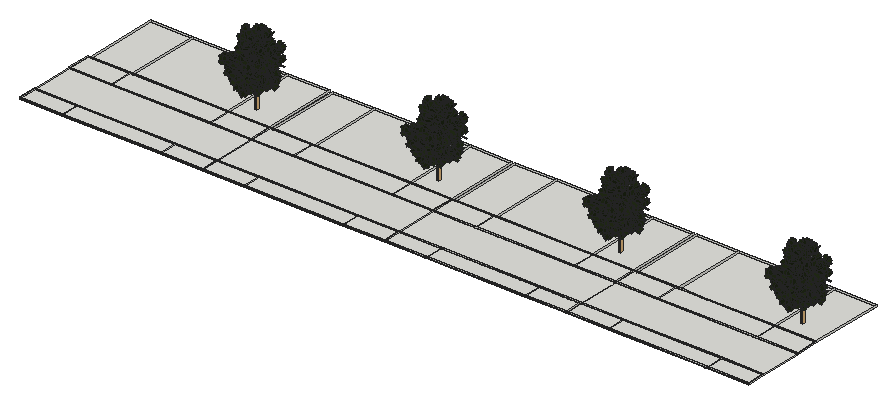
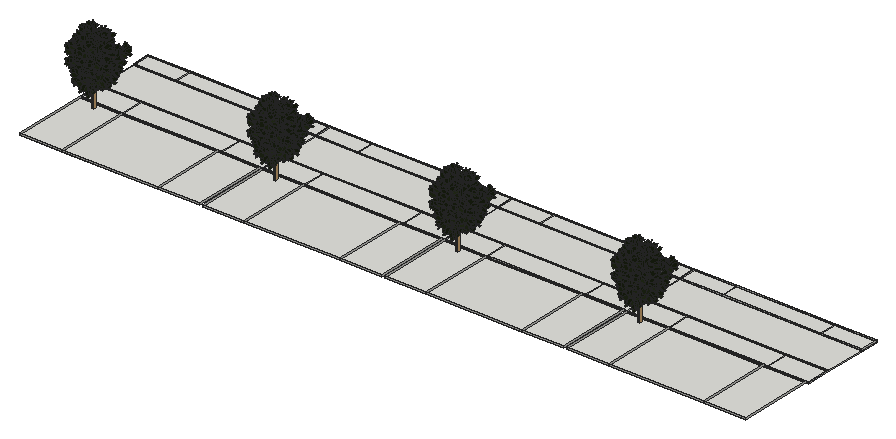
# SketchUp Ruby script. Lengths in inches.
U = 1.inch
M = Sketchup.active_model
def pt(a) = Geom::Point3d.new(a.map { |v| v * U })
def face(e, loops, mat)
  f = e.add_face(loops[0].map { |a| pt(a) })
  loops[1..].each { |l| e.add_face(l.map { |a| pt(a) }).erase! }
  f.material = f.back_material = mat if mat
  f
end
# faces: each face lists its corners as indices into pts; further lists are holes
def faces(e, pts, list, mat = nil) = list.each { |f| face(e, (f[0].is_a?(Array) ? f : [f]).map { |l| l.map { |i| pts[i] } }, mat) }
# xy, xz, yz: faces in a plane at the given z, y or x. An outline is a flat list of corners, or four numbers for a rectangle; further outlines are holes
def ring(l) = l.size == 4 ? [[l[0], l[1]], [l[2], l[1]], [l[2], l[3]], [l[0], l[3]]] : l.each_slice(2).to_a
def flat(e, list, mat, &to3) = list.each { |f| face(e, (f[0].is_a?(Array) ? f : [f]).map { |l| ring(l).map { |u, v| to3.(u, v) } }, mat) }
def xy(e, z, list, mat = nil) = flat(e, list, mat) { |x, y| [x, y, z] }
def xz(e, y, list, mat = nil) = flat(e, list, mat) { |x, z| [x, y, z] }
def yz(e, x, list, mat = nil) = flat(e, list, mat) { |y, z| [x, y, z] }
def lines(e, pts, list) = list.each { |a, b| e.add_line(pt(pts[a]), pt(pts[b])) }
# prism: a flat outline (further loops are holes) pulled along v
def prism(e, loops, v, mat = nil)
  f = face(e, loops, mat); d = Geom::Vector3d.new(v.map { |x| x * U })
  f.pushpull(f.normal.samedirection?(d) ? d.length : -d.length)
end
def box(e, o, s, mat = nil) = prism(e, [[o, [o[0] + s[0], o[1], o[2]], [o[0] + s[0], o[1] + s[1], o[2]], [o[0], o[1] + s[1], o[2]]]], [0, 0, s[2]], mat)
def at(x, y, z, deg = 0) = Geom::Transformation.translation(pt([x, y, z])) * Geom::Transformation.rotation(ORIGIN, Z_AXIS, deg.degrees)
def axes(o, x, y, z) = Geom::Transformation.new([*x, 0, *y, 0, *z, 0, *pt(o).to_a, 1])
def part(name) = M.definitions.add(name)
# library, detail: a bought-in or finely detailed component or shape, given as its bounding box
def library(name, o, s) = part(name).tap { |d| box(d.entities, o, s) }
def detail(e, o, s) = box(e.add_group.entities, o, s)
def put(e, d, t, mat = nil) = e.add_instance(d, t).tap { |i| i.material = mat if mat }
def group(e, t, mat = nil) = e.add_group.tap { |g| g.transformation = t; g.material = mat if mat }.entities
root = M.entities
M.materials.add("Green ash – green texture").color = [33, 41, 22]
M.materials.add("[Color_005]").color = [114, 114, 114]
M.materials.add("[Color_D09]1").color = [86, 59, 49]
c1 = part("Component\#31")
xz(c1.entities,0,[[2.54,0,9.87,0.64,10.99,2.07,11.4,3.42,15.13,2.28,14.48,4.31,16.14,5.21,16.14,6.08,19.81,7.28,19.6,9.67,17.45,11.49,17.45,12.16,18.82,14.37,17.48,14.37,14.41,13.66,14.41,15.23,12.5625,17.49,9.84,15.21,8.9,13.85,7.74,13.625,7.35,12.68,6.87,13.02,6.35,12.27,5.92,10.47,4.2,7.42,2.84,6.89,0,2.38,0.07,1.59,2.8125,4.94,3.37,3.59,2.54,3.37,2.12,2.22]],"Green ash – green texture")
c2 = part("Component\#30")
xz(c2.entities,0,[[1.1,0,1.61,0,2.73,1.11,4.34,2.72,5.21,6.36,5.85,7.16,6.35,6.9375,6.85,8.05,8.03,8.05,8.625,9.25,10.11,11.7,9.56,13.83,9.56,15.84,7.83,15.84,6.03,14.37,5.31,16.54,4.4375,17.39,1.45,14.31,0,9.15,1.4,5.18,3.01,6.08,1.98,1.39]],"Green ash – green texture")
c3 = part("Component\#32")
put(c3.entities,c1,axes([0,7.77,0],[1,0,0],[0,0.89571,0.44464],[0,-0.44464,0.89571]))
put(c3.entities,c2,axes([2.15,6.37,5.26],[0.57629,-0.80824,0.12095],[0.79263,0.51673,-0.3236],[0.19905,0.28236,0.93843]))
c4 = part("Component\#33")
put(c4.entities,c3,axes([-4.97,-3.22,4.05],[0.69883,-0.69034,0.18725],[0.53248,0.3273,-0.7806],[0.47759,0.64522,0.59632]))
c5 = part("Component\#34")
put(c5.entities,c4,axes([0,5.2,2.2],[1,0,0],[0,0.90259,0.43051],[0,-0.43051,0.90259]))
c6 = part("leaf group 2")
put(c6.entities,c5,axes([-11.99,4.41,-4.35],[2.22014,-0.82385,1.14017],[1.36501,1.77637,-1.37441],[-0.33979,1.75315,1.92841]))
c7 = part("Component\#37")
put(c7.entities,c6,axes([-5.27,11.65,1.68],[-0.48323,0.10636,-0.43072],[-0.11515,-0.64511,-0.03012],[-0.42845,0.05342,0.49388]))
c8 = part("Component\#36")
xz(c8.entities,0,[[0.64,0,0,0.1875,4.21,2.81,8.59,4.11,12.8,4.11,19.57,2.81,12.8,3.73,8.59,3.73,4.21,2.3125]],"[Color_D09]1")
c9 = part("Leaf cluster \#1")
put(c9.entities,c7,axes([23.53,12.57,24.85],[0.06536,-0.90475,-0.42089],[0.61791,-0.2945,0.72901],[-0.78353,-0.30772,0.53981]))
put(c9.entities,c7,axes([22.7,12.25,24.83],[-0.47146,-0.89493,0.11311],[0.80135,-0.48549,-0.35888],[0.36776,-0.0521,0.90651]))
put(c9.entities,c7,axes([24.25,0.65,20.83],[0.8253,-0.50372,0.24924],[0.23848,0.71461,0.65749],[-0.51157,-0.48438,0.71194]))
put(c9.entities,c7,axes([23.54,-2.45,18.63],[0.04689,-0.92492,0.3511],[0.72122,-0.28285,-0.64421],[0.71641,0.2674,0.65188]))
put(c9.entities,c7,axes([22.39,16.15,27.04],[-0.5311,-0.82173,0.2419],[0.41574,0.01583,0.89559],[-0.77461,0.50499,0.40813]))
put(c9.entities,c8,axes([22.76,-5.09,13.48],[0,1.66539,0.44624],[-1.72414,0,0],[0,-0.44624,1.66539]))
c10 = part("Component\#35")
p = [[0,0,0.13],[0.41,0.77,0],[4.07,2.79,10.125],[3.73,2.15,10.23],[7.66,4.77,23.875],[7.4,4.27,23.96],
  [8.6875,5.26,35.99],[8.5,4.91,36.05],[8.32,4.9375,46.95],[8.21,4.74,46.98]]
faces(c10.entities,p,[[0,1,2,3],[3,2,4,5],[4,6,7,5],[6,8,9,7]],"[Color_005]")
c11 = part("Component\#39")
put(c11.entities,c10,axes([3.13,0.17,-0.45],[3.38032,6.88592,0.52481],[-5.85488,3.97559,0.303],[0,-1.35912,3.54524]))
put(c11.entities,c7,axes([0.37,31.375,148.94],[0.47772,0.64064,-1.51139],[2.85768,-0.62659,0.20284],[-0.43926,-3.3797,-0.3241]))
c12 = part("Leafy branch \#1")
put(c12.entities,c9,axes([28.11,72.66,46.26],[0.77413,-0.41274,-0.47998],[0.6311,0.56229,0.53435],[0.04934,-0.71657,0.69577]))
put(c12.entities,c9,axes([31.25,3.94,9.17],[0.73236,0.67893,0.05208],[-0.46223,0.55185,-0.69413],[-0.5,0.48428,0.71797]))
put(c12.entities,c9,axes([20.16,84.84,57.95],[0.96628,0.19619,0.16678],[-0.2575,0.73909,0.62245],[-0.00115,-0.6444,0.76469]))
put(c12.entities,c9,axes([30.13,29.18,11.93],[0.86603,0.2796,0.41452],[0,0.82904,-0.55919],[-0.5,0.48428,0.71797]))
put(c12.entities,c9,axes([47.67,28.63,-3.7],[0.1205,-0.71255,0.69119],[0.96646,0.24327,0.08231],[-0.2268,0.65809,0.71797]))
put(c12.entities,c9,axes([48.76,50.64,76.31],[-0.6716,0.46861,-0.57389],[0.01402,0.78248,0.62252],[0.74078,0.41004,-0.53209]))
put(c12.entities,c11,axes([42.34,0,10.34],[0.39368,0,0],[0,0.22544,-0.24092],[0,0.54032,0.50562]))
put(c12.entities,c9,axes([64.51,80.82,101.08],[-0.99604,0.06562,-0.06004],[-0.0106,0.58266,0.81265],[0.08831,0.81006,-0.57966]))
c13 = library("Component\#40",[-6.35,9.4375,-76.57],[12.56,13.68,315.77])
c14 = part("Component\#43")
put(c14.entities,c9,axes([-3.64,36.17,23.18],[0.95801,0.10249,0.26779],[-0.28581,0.41631,0.86313],[-0.02302,-0.90343,0.42812]))
put(c14.entities,c9,axes([13.16,55.79,39.92],[0.70711,-0.61725,0.34497],[0,0.48786,0.87292],[-0.70711,-0.61725,0.34497]))
put(c14.entities,c11,axes([18.8125,5.17,0.46],[0.25503,0,0],[0,0.20007,-0.0752],[0,0.16866,0.44872]))
put(c14.entities,c9,axes([23.62,-10.17,21.5],[-0.56253,0.81775,0.12181],[0.38738,0.13053,0.91263],[0.73041,0.56057,-0.39021]))
put(c14.entities,c9,axes([45.18,27.18,68.96],[-0.96593,-0.22593,0.12627],[0.12295,0.02876,0.992],[-0.22775,0.97372,0]))
c15 = part("Component\#42")
put(c15.entities,c11,axes([21.47,3.93,0.22],[0.25503,0,0],[0,0.21068,-0.03601],[0,0.08077,0.47252]))
put(c15.entities,c9,axes([-4.05,13.6875,55.34],[0.70711,0.70373,-0.069],[0,0.09758,0.99523],[0.70711,-0.70373,0.069]))
put(c15.entities,c9,axes([6.52,33.54,18.07],[0.92587,-0.37604,0.03687],[0,0.09758,0.99523],[-0.37784,-0.92145,0.09035]))
c16 = part("Component\#46")
put(c16.entities,c9,axes([26.17,74.02,40.56],[0.25882,-0.64004,0.72344],[0,0.74896,0.66262],[-0.96593,-0.1715,0.19384]))
put(c16.entities,c9,axes([6.38,24.03,55.81],[-0.04786,0.8645,-0.50035],[0.15558,0.50126,0.85119],[0.98666,-0.03711,-0.15849]))
put(c16.entities,c11,axes([17.68,0,1.01],[0.32282,0,0],[0,0.21407,-0.16545],[0,0.37107,0.48011]))
put(c16.entities,c9,axes([-9.1875,31.15,28.07],[0.82314,0.37626,-0.42529],[0,0.74896,0.66262],[0.56784,-0.54543,0.61649]))
put(c16.entities,c9,axes([0.54,-12.07,9.94],[0.19622,0.90478,-0.37799],[-0.67396,0.40444,0.61823],[0.71224,0.13344,0.68914]))
put(c16.entities,c9,axes([7.34,9.15,39.57],[0.05153,0.73872,-0.67204],[0.38679,0.60565,0.6954],[0.92072,-0.29578,-0.25452]))
put(c16.entities,c9,axes([36.2,51.23,15.73],[-0.18626,-0.35374,0.91661],[-0.31641,0.90483,0.2849],[-0.93016,-0.23696,-0.28046]))
c17 = part("Tree")
put(c17.entities,c12,axes([-22.29,52.36,216.76],[0.38964,-1.07313,-0.10036],[1.06809,0.37236,0.19631],[-0.13881,-0.14712,1.22884]))
put(c17.entities,c12,axes([59.83,6.78,230.57],[-1.28826,-0.23008,-0.3647],[0.05148,-1.22938,0.51215],[-0.34663,0.55136,1.25774]))
put(c17.entities,c13,axes([-2.16,-18.04,104.22],[1.30157,0,0],[0,1.30157,0],[0,0,1.36111]))
put(c17.entities,c12,axes([-55.8,4.2,115.32],[1.30157,0,0],[0,1.29536,0.19359],[0,-0.26855,1.38538]))
put(c17.entities,c12,axes([5.36,-52.22,156.04],[-0.23532,1.19719,-0.71362],[-1.32974,0,0.39335],[0.40758,0.6912,1.23603]))
put(c17.entities,c14,axes([-20.09,22.57,317.7],[0,-1.33697,0],[1.33697,0,0],[0,0,1.4573]))
put(c17.entities,c12,axes([44.2,-31.84,172.82],[-1.11894,0.85085,0],[-0.85085,-1.11894,0],[0,0,1.53221]))
put(c17.entities,c12,axes([-10.2,63.7,119.93],[0.28716,-1.46366,0],[1.41378,0.27737,0.38604],[-0.41292,-0.08101,1.5704]))
put(c17.entities,c12,axes([-29.03,-40.72,232.79],[0.5211,0.98898,-0.38718],[-1.02974,0.58664,0.11255],[0.35577,0.28216,1.19957]))
put(c17.entities,c12,axes([44.92,21.7,135.38],[-1.05627,-0.44294,0],[0.44294,-1.05627,0],[0,0,1.24847]))
put(c17.entities,c14,axes([-32.94,-0.59,304.82],[1.2814,-0.22825,0],[0.22825,1.2814,0],[0,0,1.41871]))
put(c17.entities,c14,axes([0.6,-31.29,315.98],[0.13082,1.33422,0],[-1.33422,0.13082,0],[0,0,1.46127]))
put(c17.entities,c14,axes([21.3,1.66,315.16],[-1.25722,0.32198,-0.09905],[-0.32539,-1.26867,0.00612],[-0.08719,0.09194,1.40547]))
put(c17.entities,c15,axes([-19,30.84,372.72],[0.65078,-1.12719,0],[1.12719,0.65078,0],[0,0,1.41871]))
put(c17.entities,c15,axes([14.39,-16.125,357],[-0.73695,1.06095,0.15933],[-1.03698,-0.75397,0.2242],[0.29981,0,1.38667]))
put(c17.entities,c16,axes([-5.9,-20.03,270.39],[0,1.47598,0],[-1.4157,0,0.41751],[0.45509,0,1.54311]))
put(c17.entities,c16,axes([-18.4375,22.18,263.88],[0.84243,-1.42226,-0.32685],[1.40385,0.7063,0.64743],[-0.37678,-0.54841,1.68147]))
put(c17.entities,c16,axes([-29.32,4.9,283.41],[1.35363,0,0],[0,1.33841,0.20242],[0,-0.22063,1.45887]))
put(c17.entities,c16,axes([17.31,11.65,257.52],[-1.14969,-0.5642,-0.25322],[0.46017,-1.12719,0.50159],[-0.40066,0.32434,1.3027]))
put(c17.entities,c16,axes([16.3,15.3125,240.45],[-0.98541,-0.85203,0.68095],[1.00747,-1.01506,0.22317],[0.31818,0.5753,1.40228]))
put(c17.entities,c12,axes([-46.75,22.93,206.12],[1.08363,-0.37101,0],[0.37101,1.08363,0],[0,0,1.24847]))
put(c17.entities,c12,axes([41.1,-35.18,99.125],[-1.05556,0.85173,0.25344],[-0.84493,-1.04965,0.12953],[0.39153,-0.09409,1.38106]))
xy(root,-33.25,[[26.62,0,313.69,126.25],[313.69,0,990.19,126.25],[990.19,0,1277.25,126.25],[1277.25,0,1564.31,126.25],[1564.31,0,2240.81,126.25],
  [2240.81,0,2527.87,126.25],[2527.87,0,2814.94,126.25],[2814.94,0,3491.44,126.25],[3491.44,0,3778.5,126.25],[3778.5,0,4065.56,126.25],
  [4065.56,0,4742.06,126.25],[4742.06,0,5029.12,126.25],[26.62,126.25,313.69,419.4375],[313.69,126.25,990.19,419.4375],[990.19,126.25,1277.25,419.4375],
  [1277.25,126.25,1564.31,419.4375],[1564.31,126.25,2240.81,419.4375],[2240.81,126.25,2527.87,419.4375],[2527.87,126.25,2814.94,419.4375],[2814.94,126.25,3491.44,419.4375],
  [3491.44,126.25,3778.5,419.4375],[3778.5,126.25,4065.56,419.4375],[4065.56,126.25,4742.06,419.4375],[4742.06,126.25,5029.12,419.4375],[26.62,419.4375,313.69,581.125],
  [313.69,419.4375,990.19,581.125],[990.19,419.4375,1277.25,581.125],[1277.25,419.4375,1564.31,581.125],[1564.31,419.4375,2240.81,581.125],[2240.81,419.4375,2527.87,581.125],
  [2527.87,419.4375,2814.94,581.125],[2814.94,419.4375,3491.44,581.125],[3491.44,419.4375,3778.5,581.125],[3778.5,419.4375,4065.56,581.125],[4065.56,419.4375,4742.06,581.125],
  [4742.06,419.4375,5029.12,581.125],[46.37,581.125,333.44,1096.5],[333.44,581.125,990.19,1096.5],[990.19,581.125,1277.25,1096.5],[1297,581.125,1584.06,1096.5],
  [1584.06,581.125,2240.81,1096.5],[2240.81,581.125,2527.87,1096.5],[2547.62,581.125,2834.69,1096.5],[2834.69,581.125,3491.44,1096.5],[3491.44,581.125,3778.5,1096.5],
  [3798.25,581.125,4085.31,1096.5],[4085.31,581.125,4742.06,1096.5],[4742.06,581.125,5029.12,1096.5]])
xy(root,-27.3125,[[26.62,0,313.69,126.25],[313.69,0,990.19,126.25],[990.19,0,1277.25,126.25],[1277.25,0,1564.31,126.25],[1564.31,0,2240.81,126.25],
  [2240.81,0,2527.87,126.25],[2527.87,0,2814.94,126.25],[2814.94,0,3491.44,126.25],[3491.44,0,3778.5,126.25],[3778.5,0,4065.56,126.25],
  [4065.56,0,4742.06,126.25],[4742.06,0,5029.12,126.25],[26.62,126.25,1277.25,419.4375],[1277.25,126.25,2527.87,419.4375],[2527.87,126.25,3778.5,419.4375],
  [3778.5,126.25,5029.12,419.4375],[26.62,419.4375,313.69,581.125],[313.69,419.4375,990.19,581.125],[990.19,419.4375,1277.25,581.125],[1277.25,419.4375,1564.31,581.125],
  [1564.31,419.4375,2240.81,581.125],[2240.81,419.4375,2527.87,581.125],[2527.87,419.4375,2814.94,581.125],[2814.94,419.4375,3491.44,581.125],[3491.44,419.4375,3778.5,581.125],
  [3778.5,419.4375,4065.56,581.125],[4065.56,419.4375,4742.06,581.125],[4742.06,419.4375,5029.12,581.125]])
xz(root,0,[[26.62,-33.25,313.69,-27.3125],[313.69,-33.25,990.19,-27.3125],[990.19,-33.25,1277.25,-27.3125],[1277.25,-33.25,1564.31,-27.3125],[1564.31,-33.25,2240.81,-27.3125],
  [2240.81,-33.25,2527.87,-27.3125],[2527.87,-33.25,2814.94,-27.3125],[2814.94,-33.25,3491.44,-27.3125],[3491.44,-33.25,3778.5,-27.3125],[3778.5,-33.25,4065.56,-27.3125],
  [4065.56,-33.25,4742.06,-27.3125],[4742.06,-33.25,5029.12,-27.3125],[26.62,-27.3125,313.69,-20.25],[313.69,-27.3125,990.19,-20.25],[990.19,-27.3125,1277.25,-20.25],
  [1277.25,-27.3125,1564.31,-20.25],[1564.31,-27.3125,2240.81,-20.25],[2240.81,-27.3125,2527.87,-20.25],[2527.87,-27.3125,2814.94,-20.25],[2814.94,-27.3125,3491.44,-20.25],
  [3491.44,-27.3125,3778.5,-20.25],[3778.5,-27.3125,4065.56,-20.25],[4065.56,-27.3125,4742.06,-20.25],[4742.06,-27.3125,5029.12,-20.25]])
xz(root,126.25,[[26.62,-33.25,313.69,-27.3125],[313.69,-33.25,990.19,-27.3125],[990.19,-33.25,1277.25,-27.3125],[1277.25,-33.25,1564.31,-27.3125],[1564.31,-33.25,2240.81,-27.3125],
  [2240.81,-33.25,2527.87,-27.3125],[2527.87,-33.25,2814.94,-27.3125],[2814.94,-33.25,3491.44,-27.3125],[3491.44,-33.25,3778.5,-27.3125],[3778.5,-33.25,4065.56,-27.3125],
  [4065.56,-33.25,4742.06,-27.3125],[4742.06,-33.25,5029.12,-27.3125],[26.62,-27.3125,313.69,-20.25],[313.69,-27.3125,990.19,-20.25],[990.19,-27.3125,1277.25,-20.25],
  [1277.25,-27.3125,1564.31,-20.25],[1564.31,-27.3125,2240.81,-20.25],[2240.81,-27.3125,2527.87,-20.25],[2527.87,-27.3125,2814.94,-20.25],[2814.94,-27.3125,3491.44,-20.25],
  [3491.44,-27.3125,3778.5,-20.25],[3778.5,-27.3125,4065.56,-20.25],[4065.56,-27.3125,4742.06,-20.25],[4742.06,-27.3125,5029.12,-20.25]])
xz(root,419.4375,[[26.62,-33.25,313.69,-27.3125],[313.69,-33.25,990.19,-27.3125],[990.19,-33.25,1277.25,-27.3125],[1277.25,-33.25,1564.31,-27.3125],[1564.31,-33.25,2240.81,-27.3125],
  [2240.81,-33.25,2527.87,-27.3125],[2527.87,-33.25,2814.94,-27.3125],[2814.94,-33.25,3491.44,-27.3125],[3491.44,-33.25,3778.5,-27.3125],[3778.5,-33.25,4065.56,-27.3125],
  [4065.56,-33.25,4742.06,-27.3125],[4742.06,-33.25,5029.12,-27.3125],[26.62,-27.3125,313.69,-20.5],[313.69,-27.3125,990.19,-20.5],[990.19,-27.3125,1277.25,-20.5],
  [1277.25,-27.3125,1564.31,-20.5],[1564.31,-27.3125,2240.81,-20.5],[2240.81,-27.3125,2527.87,-20.5],[2527.87,-27.3125,2814.94,-20.5],[2814.94,-27.3125,3491.44,-20.5],
  [3491.44,-27.3125,3778.5,-20.5],[3778.5,-27.3125,4065.56,-20.5],[4065.56,-27.3125,4742.06,-20.5],[4742.06,-27.3125,5029.12,-20.5]])
xz(root,581.125,[[26.62,-33.25,46.37,-27.3125],[46.37,-33.25,313.69,-27.3125],[313.69,-33.25,333.44,-27.3125],[333.44,-33.25,492.21,-27.3125],[492.21,-33.25,527.2,-27.3125],
  [527.2,-33.25,939.09,-27.3125],[939.09,-33.25,990.19,-27.3125],[990.19,-33.25,1277.25,-27.3125],[1277.25,-33.25,1297,-27.3125],[1297,-33.25,1564.31,-27.3125],
  [1564.31,-33.25,1584.06,-27.3125],[1584.06,-33.25,1742.84,-27.3125],[1742.84,-33.25,1777.83,-27.3125],[1777.83,-33.25,2189.71,-27.3125],[2189.71,-33.25,2240.81,-27.3125],
  [2240.81,-33.25,2527.87,-27.3125],[2527.87,-33.25,2547.62,-27.3125],[2547.62,-33.25,2814.94,-27.3125],[2814.94,-33.25,2834.69,-27.3125],[2834.69,-33.25,2993.46,-27.3125],
  [2993.46,-33.25,3028.45,-27.3125],[3028.45,-33.25,3440.34,-27.3125],[3440.34,-33.25,3491.44,-27.3125],[3491.44,-33.25,3778.5,-27.3125],[3778.5,-33.25,3798.25,-27.3125],
  [3798.25,-33.25,4065.56,-27.3125],[4065.56,-33.25,4085.31,-27.3125],[4085.31,-33.25,4244.09,-27.3125],[4244.09,-33.25,4279.08,-27.3125],[4279.08,-33.25,4690.96,-27.3125],
  [4690.96,-33.25,4742.06,-27.3125],[4742.06,-33.25,5029.12,-27.3125],[26.62,-27.3125,46.37,-20.5],[46.37,-27.3125,313.69,-20.5],[313.69,-27.3125,333.44,-20.5],
  [333.44,-27.3125,492.21,-20.5],[492.21,-27.3125,527.2,-20.5],[527.2,-27.3125,939.09,-20.5],[939.09,-27.3125,990.19,-20.5],[990.19,-27.3125,1277.25,-20.5],
  [1277.25,-27.3125,1297,-20.5],[1297,-27.3125,1564.31,-20.5],[1564.31,-27.3125,1584.06,-20.5],[1584.06,-27.3125,1742.84,-20.5],[1742.84,-27.3125,1777.83,-20.5],
  [1777.83,-27.3125,2189.71,-20.5],[2189.71,-27.3125,2240.81,-20.5],[2240.81,-27.3125,2527.87,-20.5],[2527.87,-27.3125,2547.62,-20.5],[2547.62,-27.3125,2814.94,-20.5],
  [2814.94,-27.3125,2834.69,-20.5],[2834.69,-27.3125,2993.46,-20.5],[2993.46,-27.3125,3028.45,-20.5],[3028.45,-27.3125,3440.34,-20.5],[3440.34,-27.3125,3491.44,-20.5],
  [3491.44,-27.3125,3778.5,-20.5],[3778.5,-27.3125,3798.25,-20.5],[3798.25,-27.3125,4065.56,-20.5],[4065.56,-27.3125,4085.31,-20.5],[4085.31,-27.3125,4244.09,-20.5],
  [4244.09,-27.3125,4279.08,-20.5],[4279.08,-27.3125,4690.96,-20.5],[4690.96,-27.3125,4742.06,-20.5],[4742.06,-27.3125,5029.12,-20.5]])
xz(root,1096.5,[[46.37,-33.25,333.44,-20.5],[333.44,-33.25,990.19,-20.5],[990.19,-33.25,1277.25,-20.5],[1297,-33.25,1584.06,-20.5],[1584.06,-33.25,2240.81,-20.5],
  [2240.81,-33.25,2527.87,-20.5],[2547.62,-33.25,2834.69,-20.5],[2834.69,-33.25,3491.44,-20.5],[3491.44,-33.25,3778.5,-20.5],[3798.25,-33.25,4085.31,-20.5],
  [4085.31,-33.25,4742.06,-20.5],[4742.06,-33.25,5029.12,-20.5]])
yz(root,26.62,[[0,-33.25,126.25,-27.3125],[126.25,-33.25,419.4375,-27.3125],[419.4375,-33.25,581.125,-27.3125],[0,-27.3125,126.25,-20.25],[419.4375,-27.3125,581.125,-20.5]])
yz(root,46.37,[[581.125,-33.25,1096.5,-20.5]])
yz(root,313.69,[[0,-33.25,126.25,-27.3125],[419.4375,-33.25,581.125,-27.3125]])
yz(root,333.44,[[581.125,-33.25,1096.5,-20.5]])
yz(root,990.19,[[0,-33.25,126.25,-27.3125],[419.4375,-33.25,581.125,-27.3125],[581.125,-33.25,1096.5,-20.5]])
yz(root,1277.25,[[0,-33.25,126.25,-27.3125],[126.25,-33.25,419.4375,-27.3125],[419.4375,-33.25,581.125,-27.3125],[581.125,-33.25,1096.5,-20.5],[0,-27.3125,126.25,-20.25],
  [419.4375,-27.3125,581.125,-20.5]])
yz(root,1297,[[581.125,-33.25,1096.5,-20.5]])
yz(root,1564.31,[[0,-33.25,126.25,-27.3125],[419.4375,-33.25,581.125,-27.3125]])
yz(root,1584.06,[[581.125,-33.25,1096.5,-20.5]])
yz(root,2240.81,[[0,-33.25,126.25,-27.3125],[419.4375,-33.25,581.125,-27.3125],[581.125,-33.25,1096.5,-20.5]])
yz(root,2527.87,[[0,-33.25,126.25,-27.3125],[126.25,-33.25,419.4375,-27.3125],[419.4375,-33.25,581.125,-27.3125],[581.125,-33.25,1096.5,-20.5],[0,-27.3125,126.25,-20.25],
  [419.4375,-27.3125,581.125,-20.5]])
yz(root,2547.62,[[581.125,-33.25,1096.5,-20.5]])
yz(root,2814.94,[[0,-33.25,126.25,-27.3125],[419.4375,-33.25,581.125,-27.3125]])
yz(root,2834.69,[[581.125,-33.25,1096.5,-20.5]])
yz(root,3491.44,[[0,-33.25,126.25,-27.3125],[419.4375,-33.25,581.125,-27.3125],[581.125,-33.25,1096.5,-20.5]])
yz(root,3778.5,[[0,-33.25,126.25,-27.3125],[126.25,-33.25,419.4375,-27.3125],[419.4375,-33.25,581.125,-27.3125],[581.125,-33.25,1096.5,-20.5],[0,-27.3125,126.25,-20.25],
  [419.4375,-27.3125,581.125,-20.5]])
yz(root,3798.25,[[581.125,-33.25,1096.5,-20.5]])
yz(root,4065.56,[[0,-33.25,126.25,-27.3125],[419.4375,-33.25,581.125,-27.3125]])
yz(root,4085.31,[[581.125,-33.25,1096.5,-20.5]])
yz(root,4742.06,[[0,-33.25,126.25,-27.3125],[419.4375,-33.25,581.125,-27.3125],[581.125,-33.25,1096.5,-20.5]])
yz(root,5029.12,[[0,-33.25,126.25,-27.3125],[126.25,-33.25,419.4375,-27.3125],[419.4375,-33.25,581.125,-27.3125],[581.125,-33.25,1096.5,-20.5],[0,-27.3125,126.25,-20.25],
  [419.4375,-27.3125,581.125,-20.5]])
put(root,c17,at(3621.93,661.87,0))
put(root,c17,at(4872.55,661.87,0))
put(root,c17,at(1120.68,661.87,0))
put(root,c17,at(2371.3,661.87,0))
